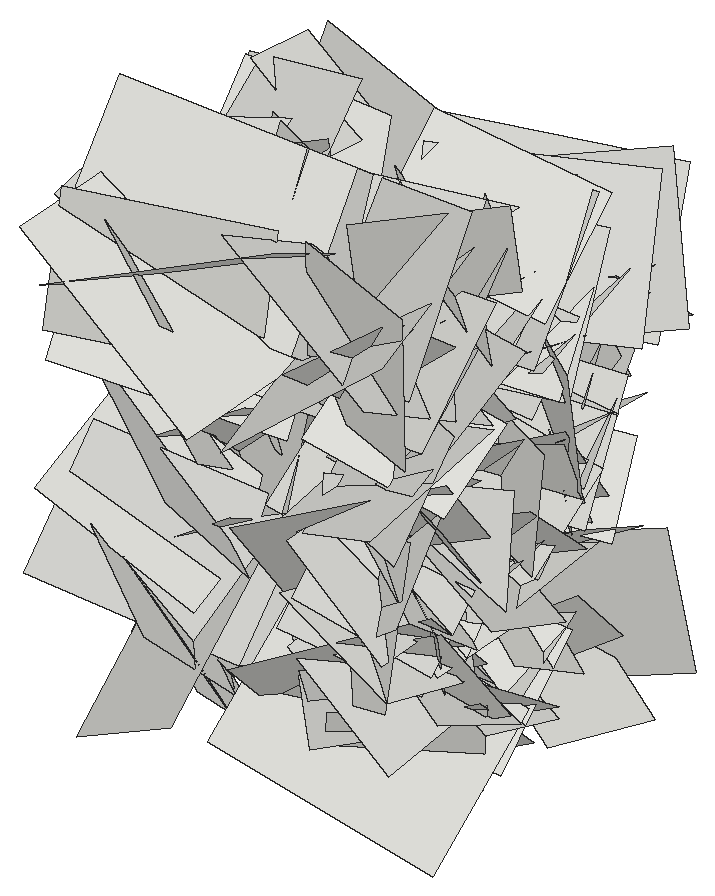
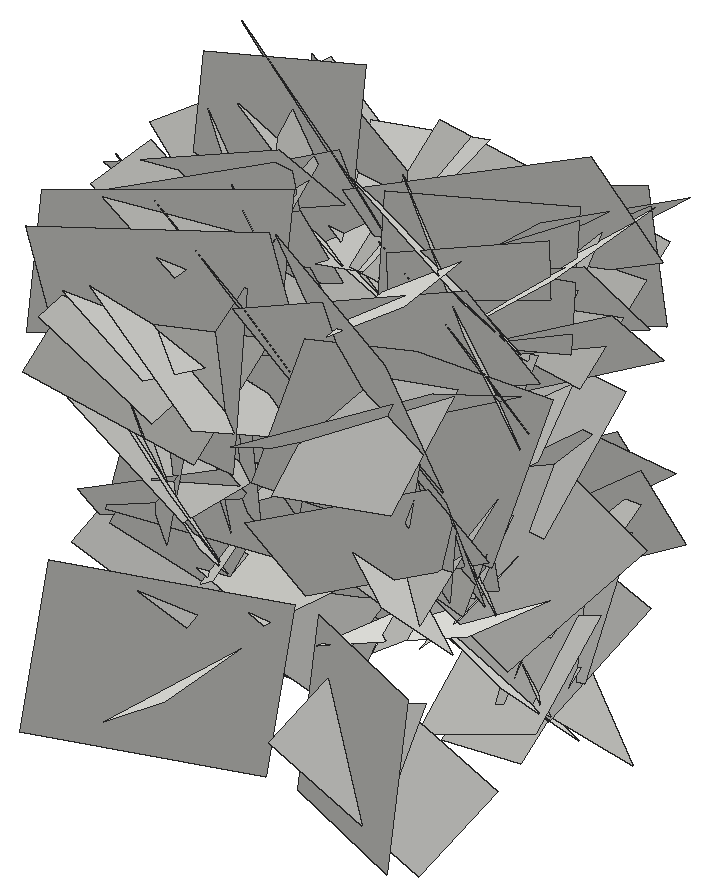
# SketchUp Ruby script. Lengths in inches.
U = 1.inch
M = Sketchup.active_model
def pt(a) = Geom::Point3d.new(a.map { |v| v * U })
def face(e, loops, mat)
  f = e.add_face(loops[0].map { |a| pt(a) })
  loops[1..].each { |l| e.add_face(l.map { |a| pt(a) }).erase! }
  f.material = f.back_material = mat if mat
  f
end
# faces: each face lists its corners as indices into pts; further lists are holes
def faces(e, pts, list, mat = nil) = list.each { |f| face(e, (f[0].is_a?(Array) ? f : [f]).map { |l| l.map { |i| pts[i] } }, mat) }
# xy, xz, yz: faces in a plane at the given z, y or x. An outline is a flat list of corners, or four numbers for a rectangle; further outlines are holes
def ring(l) = l.size == 4 ? [[l[0], l[1]], [l[2], l[1]], [l[2], l[3]], [l[0], l[3]]] : l.each_slice(2).to_a
def flat(e, list, mat, &to3) = list.each { |f| face(e, (f[0].is_a?(Array) ? f : [f]).map { |l| ring(l).map { |u, v| to3.(u, v) } }, mat) }
def xy(e, z, list, mat = nil) = flat(e, list, mat) { |x, y| [x, y, z] }
def xz(e, y, list, mat = nil) = flat(e, list, mat) { |x, z| [x, y, z] }
def yz(e, x, list, mat = nil) = flat(e, list, mat) { |y, z| [x, y, z] }
def lines(e, pts, list) = list.each { |a, b| e.add_line(pt(pts[a]), pt(pts[b])) }
# prism: a flat outline (further loops are holes) pulled along v
def prism(e, loops, v, mat = nil)
  f = face(e, loops, mat); d = Geom::Vector3d.new(v.map { |x| x * U })
  f.pushpull(f.normal.samedirection?(d) ? d.length : -d.length)
end
def box(e, o, s, mat = nil) = prism(e, [[o, [o[0] + s[0], o[1], o[2]], [o[0] + s[0], o[1] + s[1], o[2]], [o[0], o[1] + s[1], o[2]]]], [0, 0, s[2]], mat)
def at(x, y, z, deg = 0) = Geom::Transformation.translation(pt([x, y, z])) * Geom::Transformation.rotation(ORIGIN, Z_AXIS, deg.degrees)
def axes(o, x, y, z) = Geom::Transformation.new([*x, 0, *y, 0, *z, 0, *pt(o).to_a, 1])
def part(name) = M.definitions.add(name)
# library, detail: a bought-in or finely detailed component or shape, given as its bounding box
def library(name, o, s) = part(name).tap { |d| box(d.entities, o, s) }
def detail(e, o, s) = box(e.add_group.entities, o, s)
def put(e, d, t, mat = nil) = e.add_instance(d, t).tap { |i| i.material = mat if mat }
def group(e, t, mat = nil) = e.add_group.tap { |g| g.transformation = t; g.material = mat if mat }.entities
root = M.entities
c1 = part("Component\#6")
p = [[0.01,0,0],[0,3.24,4.54],[4.32,3.24,4.54],[4.33,0,0]]
faces(c1.entities,p,[[0,1,2,3]])
put(root,c1,axes([410.71,158.35,30.49],[-0.08461,0.81055,-0.03501],[-0.12527,-0.04642,-0.80528],[0.85081,0.07377,-0.12204]))
put(root,c1,axes([414.68,161.79,25.53],[-0.01152,-0.82607,0.19056],[-0.15176,0.18963,0.81386],[-0.88572,-0.02175,-0.14193]))
put(root,c1,axes([414.68,162.32,28.44],[-0.12821,-0.42216,-0.69512],[0.01339,-0.70366,0.42514],[-0.86197,0.05186,0.11]))
put(root,c1,axes([400.91,160.22,28.4],[0.15479,0.80897,-0.76348],[-0.02106,-0.76802,-0.81757],[1.17891,-0.11994,0.08565]))
put(root,c1,axes([414.68,160.22,28.4],[-0.15479,0.80897,-0.76348],[0.02106,-0.76802,-0.81757],[-1.17891,-0.11994,0.08565]))
put(root,c1,axes([410.71,158.39,26.84],[-0.02686,0.84806,0.10272],[-0.17857,0.09579,-0.83237],[0.88773,0.04493,-0.16432]))
put(root,c1,axes([400.91,158.99,33.95],[0.09747,0.08794,1.12692],[0.17247,1.11783,-0.1005],[1.18568,-0.16983,-0.07802]))
put(root,c1,axes([414.68,158.99,33.95],[-0.09747,0.08794,1.12692],[-0.17247,1.11783,-0.1005],[-1.18568,-0.16983,-0.07802]))
put(root,c1,axes([404.88,161.42,33.85],[0.12931,-0.58697,0.4315],[0.06321,0.44408,0.58723],[-0.76963,-0.06214,0.12073]))
put(root,c1,axes([410.71,161.42,33.85],[-0.12931,-0.58697,0.4315],[-0.06321,0.44408,0.58723],[0.76963,-0.06214,0.12073]))
put(root,c1,axes([400.91,158.06,26.05],[0.19995,0.52409,1.06255],[0.00833,1.07535,-0.5318],[1.25583,-0.09057,-0.16565]))
put(root,c1,axes([414.68,158.06,26.05],[-0.19995,0.52409,1.06255],[-0.00833,1.07535,-0.5318],[-1.25583,-0.09057,-0.16565]))
put(root,c1,axes([400.91,157.9,37.93],[0.24747,1.3445,0.30187],[-0.11522,0.32319,-1.35538],[1.4561,-0.20293,-0.15855]))
put(root,c1,axes([414.68,157.9,37.93],[-0.24747,1.3445,0.30187],[0.11522,0.32319,-1.35538],[-1.4561,-0.20293,-0.15855]))
put(root,c1,axes([414.68,157.3125,32.29],[0.25179,1.05256,0.51222],[-0.06429,0.53303,-1.06718],[-1.23914,0.18623,0.15945]))
put(root,c1,axes([414.68,158.45,30.92],[0.16236,0.46297,0.88251],[-0.09478,0.89566,-0.45434],[-1.05211,-0.00924,0.17712]))
put(root,c1,axes([400.91,160.96,32.62],[0.12215,0.75895,-0.88724],[0.014,-0.89234,-0.7616],[1.23753,-0.06482,0.09619]))
put(root,c1,axes([414.68,160.96,32.62],[-0.12215,0.75895,-0.88724],[-0.014,-0.89234,-0.7616],[-1.23753,-0.06482,0.09619]))
put(root,c1,axes([400.91,160.7,27.63],[-0.09928,0.64406,-0.88513],[0.13228,-0.87629,-0.65083],[1.15276,0.15602,-0.00154]))
put(root,c1,axes([414.68,160.7,27.63],[0.09928,0.64406,-0.88513],[-0.13228,-0.87629,-0.65083],[-1.15276,0.15602,-0.00154]))
put(root,c1,axes([410.71,160.06,22.6],[-0.02839,-0.24478,0.77995],[-0.15528,0.76918,0.23637],[0.85248,0.13195,0.06903]))
put(root,c1,axes([400.91,164.92,23.28],[0.02573,-1.02703,-0.88101],[-0.12942,-0.87922,1.02158],[1.42847,-0.06116,0.10843]))
put(root,c1,axes([414.68,164.92,23.28],[-0.02573,-1.02703,-0.88101],[0.12942,-0.87922,1.02158],[-1.42847,-0.06116,0.10843]))
put(root,c1,axes([410.71,159.46,22.85],[-0.09982,-0.0635,0.89488],[-0.1784,0.88507,0.04509],[0.93408,0.16225,0.10424]))
put(root,c1,axes([400.91,158.58,28.72],[0.17742,0.80309,0.64454],[-0.10421,0.66248,-0.79991],[1.08655,-0.0676,-0.18196]))
put(root,c1,axes([414.68,158.58,28.72],[-0.17742,0.80309,0.64454],[0.10421,0.66248,-0.79991],[-1.08655,-0.0676,-0.18196]))
put(root,c1,axes([414.68,162.92,24.26],[-0.16568,0.16434,-0.80239],[0.1251,-0.80382,-0.18763],[-0.85913,-0.14874,0.12742]))
put(root,c1,axes([400.91,163.2,33.68],[0.16473,-1.2102,0.57798],[0.2383,0.59712,1.18983],[1.40149,0.04071,-0.27024]))
put(root,c1,axes([414.68,163.2,33.68],[-0.16473,-1.2102,0.57798],[-0.2383,0.59712,1.18983],[-1.40149,0.04071,-0.27024]))
put(root,c1,axes([414.68,163.85,33.45],[0.03445,-0.73428,-0.4148],[-0.17499,-0.41262,0.71747],[-0.87664,0.05351,-0.15952]))
put(root,c1,axes([414.68,162.43,26.35],[-0.02315,-0.70596,0.51236],[0.01203,0.51225,0.70629],[-0.92456,0.02434,-0.00364]))
put(root,c1,axes([414.68,162.61,28.57],[0.04222,-0.49534,0.62953],[-0.20196,0.60636,0.48917],[-0.82474,-0.17384,-0.08755]))
put(root,c1,axes([410.71,162.33,29.83],[-0.22776,0.38392,-0.75072],[0.01782,-0.77261,-0.39993],[0.89361,0.11326,-0.18337]))
put(root,c1,axes([414.68,164.2,31.01],[0.06613,-0.18181,-0.96198],[-0.02897,-0.96387,0.1804],[-1.03734,0.01533,-0.06637]))
put(root,c1,axes([410.71,159.67,28.14],[-0.12868,0.67272,0.52517],[-0.08613,0.51893,-0.68352],[0.90053,0.14576,0.00967]))
put(root,c1,axes([404.88,163.13,28.77],[0.13219,-0.55975,0.33448],[0.05965,0.34851,0.56225],[-0.68862,-0.07726,0.11291]))
put(root,c1,axes([410.71,163.13,28.77],[-0.13219,-0.55975,0.33448],[-0.05965,0.34851,0.56225],[0.68862,-0.07726,0.11291]))
put(root,c1,axes([400.91,159.18,36.25],[0.04304,0.74935,1.15311],[0.14712,1.14549,-0.74928],[1.45028,-0.13844,0.04179]))
put(root,c1,axes([414.68,159.18,36.25],[-0.04304,0.74935,1.15311],[-0.14712,1.14549,-0.74928],[-1.45028,-0.13844,0.04179]))
put(root,c1,axes([410.71,164.96,33.58],[0.03363,-0.67551,-0.53197],[-0.14584,-0.52946,0.66412],[0.89967,-0.06058,0.12754]))
put(root,c1,axes([400.91,159.8,34.2],[-0.03301,0.77795,0.85676],[0.24326,0.8442,-0.75821],[1.20233,-0.14944,0.17692]))
put(root,c1,axes([414.68,159.8,34.2],[0.03301,0.77795,0.85676],[-0.24326,0.8442,-0.75821],[-1.20233,-0.14944,0.17692]))
put(root,c1,axes([414.68,164.8,26.41],[-0.06555,-0.88967,-0.10275],[0.1194,-0.1099,0.88381],[-0.94178,0.04799,0.1192]))
put(root,c1,axes([414.68,163.99,40.83],[-0.08038,0.23372,-0.81219],[0.10222,-0.80774,-0.24144],[-0.89001,-0.11388,0.04562]))
put(root,c1,axes([400.91,162.55,24.47],[0.08094,0.6993,-0.63815],[0.06519,-0.64254,-0.69674],[1.00139,-0.01469,0.09694]))
put(root,c1,axes([414.68,162.55,24.47],[-0.08094,0.6993,-0.63815],[-0.06519,-0.64254,-0.69674],[-1.00139,-0.01469,0.09694]))
put(root,c1,axes([400.91,164.67,22.86],[-0.07455,-1.03669,0.46758],[0.01691,0.46753,1.03897],[1.20537,-0.07068,0.01434]))
put(root,c1,axes([414.68,164.67,22.86],[0.07455,-1.03669,0.46758],[-0.01691,0.46753,1.03897],[-1.20537,-0.07068,0.01434]))
put(root,c1,axes([400.91,159.15,32.85],[-0.28722,0.93511,0.86971],[-0.00467,0.88838,-0.95656],[1.35365,0.20148,0.18123]))
put(root,c1,axes([414.68,159.15,32.85],[0.28722,0.93511,0.86971],[0.00467,0.88838,-0.95656],[-1.35365,0.20148,0.18123]))
put(root,c1,axes([400.91,159.57,38.3125],[-0.19748,1.37219,0.09956],[-0.15298,0.08042,-1.37849],[1.4503,0.19533,-0.13185]))
put(root,c1,axes([414.68,159.57,38.3125],[0.19748,1.37219,0.09956],[0.15298,0.08042,-1.37849],[-1.4503,0.19533,-0.13185]))
put(root,c1,axes([404.88,163.1,21.29],[0.03251,-0.459,0.52355],[0.17075,0.51451,0.44164],[-0.71801,0.10157,0.12873]))
put(root,c1,axes([410.71,163.1,21.29],[-0.03251,-0.459,0.52355],[-0.17075,0.51451,0.44164],[0.71801,0.10157,0.12873]))
put(root,c1,axes([400.91,162.15,25.43],[-0.09766,0.84172,-0.54191],[0.18116,-0.52299,-0.84139],[1.04557,0.16923,0.09516]))
put(root,c1,axes([414.68,162.15,25.43],[0.09766,0.84172,-0.54191],[-0.18116,-0.52299,-0.84139],[-1.04557,0.16923,0.09516]))
put(root,c1,axes([404.88,163.79,31.02],[0.0186,-0.39942,0.51021],[0.04828,0.50989,0.39761],[-0.68514,0.02509,0.04187]))
put(root,c1,axes([410.71,163.79,31.02],[-0.0186,-0.39942,0.51021],[-0.04828,0.50989,0.39761],[0.68514,0.02509,0.04187]))
put(root,c1,axes([400.91,166.67,25.47],[-0.29316,-1.18227,0.54308],[0.10516,0.53443,1.21398],[1.37509,-0.29293,0.02294]))
put(root,c1,axes([414.68,166.67,25.47],[0.29316,-1.18227,0.54308],[-0.10516,0.53443,1.21398],[-1.37509,-0.29293,0.02294]))
put(root,c1,axes([400.91,166.97,25.06],[-0.03339,-0.82276,-0.77538],[0.30966,-0.75526,0.78954],[1.15769,0.17829,-0.23355]))
put(root,c1,axes([414.68,166.97,25.06],[0.03339,-0.82276,-0.77538],[-0.30966,-0.75526,0.78954],[-1.15769,0.17829,-0.23355]))
put(root,c1,axes([400.91,163.625,35.04],[0.27654,-0.44632,0.88094],[-0.09901,0.89592,0.48157],[1.04211,0.20356,-0.18801]))
put(root,c1,axes([414.68,163.625,35.04],[-0.27654,-0.44632,0.88094],[0.09901,0.89592,0.48157],[-1.04211,0.20356,-0.18801]))
put(root,c1,axes([414.68,166.33,22.3],[0.05809,-0.87115,0.26873],[-0.09257,0.26296,0.87026],[-0.96191,-0.07791,-0.06752]))
put(root,c1,axes([400.91,168.45,29.92],[0.2904,-0.81126,-1.09363],[-0.15157,-1.12651,0.79984],[1.4354,0.04517,0.30571]))
put(root,c1,axes([414.68,168.45,29.92],[-0.2904,-0.81126,-1.09363],[0.15157,-1.12651,0.79984],[-1.4354,0.04517,0.30571]))
put(root,c1,axes([404.88,165.16,26.22],[-0.00662,-0.41647,0.48084],[0.04981,0.47925,0.41571],[-0.67246,0.0396,0.02606]))
put(root,c1,axes([410.71,165.16,26.22],[0.00662,-0.41647,0.48084],[-0.04981,0.47925,0.41571],[0.67246,0.0396,0.02606]))
put(root,c1,axes([404.88,165.91,24.52],[-0.03596,-0.58924,0.24858],[0.15481,0.23521,0.57749],[-0.65999,0.08727,0.12191]))
put(root,c1,axes([410.71,165.91,24.52],[0.03596,-0.58924,0.24858],[-0.15481,0.23521,0.57749],[0.65999,0.08727,0.12191]))
put(root,c1,axes([404.88,167.47,38.84],[0.19203,-0.25676,-0.78485],[0.09527,-0.79261,0.28005],[-0.87013,-0.14344,-0.14255]))
put(root,c1,axes([410.71,167.47,38.84],[-0.19203,-0.25676,-0.78485],[-0.09527,-0.79261,0.28005],[0.87013,-0.14344,-0.14255]))
put(root,c1,axes([400.91,168.75,37.98],[-0.06882,-0.53698,-1.12739],[-0.1022,-1.12338,0.54063],[1.31971,-0.115,-0.01692]))
put(root,c1,axes([414.68,168.75,37.98],[0.06882,-0.53698,-1.12739],[0.1022,-1.12338,0.54063],[-1.31971,-0.115,-0.01692]))
put(root,c1,axes([414.68,164.95,29.96],[0.04265,0.57286,-0.52342],[-0.15347,-0.50938,-0.56862],[-0.80809,0.12697,0.08036]))
put(root,c1,axes([414.68,167.29,35.58],[-0.17595,-0.29467,-0.74084],[-0.05215,-0.7515,0.30993],[-0.84352,0.10793,0.13537]))
put(root,c1,axes([410.71,167.69,34.89],[0.01272,-0.59445,-0.3878],[0.01652,-0.38754,0.59453],[0.75216,0.01856,-0.0065]))
put(root,c1,axes([414.68,168.37,37.02],[0.06582,-0.55881,-0.84289],[-0.17414,-0.83883,0.54402],[-1.05774,0.10333,-0.14201]))
put(root,c1,axes([400.91,168.37,37.02],[-0.06582,-0.55881,-0.84289],[0.17414,-0.83883,0.54402],[1.05774,0.10333,-0.14201]))
put(root,c1,axes([400.91,163.85,26.9],[0.03329,1.04875,0.11229],[0.24045,0.10299,-1.02538],[1.09187,-0.05466,0.22238]))
put(root,c1,axes([414.68,163.85,26.9],[-0.03329,1.04875,0.11229],[-0.24045,0.10299,-1.02538],[-1.09187,-0.05466,0.22238]))
put(root,c1,axes([410.71,168.18,25.35],[0.0356,-0.79141,-0.13903],[-0.13499,-0.14264,0.78117],[0.84098,0.01061,0.13127]))
put(root,c1,axes([414.68,164.5,23.79],[-0.04443,0.667,0.37408],[-0.11412,0.36576,-0.66423],[-0.80255,-0.08894,0.07374]))
put(root,c1,axes([400.91,166.55,31.56],[0.0814,0.41102,-0.8284],[0.17089,-0.82447,-0.39413],[0.96524,0.11131,0.13964]))
put(root,c1,axes([414.68,166.55,31.56],[-0.0814,0.41102,-0.8284],[-0.17089,-0.82447,-0.39413],[-0.96524,0.11131,0.13964]))
put(root,c1,axes([400.91,166.62,31.96],[0.21061,0.75098,-0.921],[-0.02022,-0.93165,-0.76377],[1.25951,-0.14053,0.14175]))
put(root,c1,axes([414.68,166.62,31.96],[-0.21061,0.75098,-0.921],[0.02022,-0.93165,-0.76377],[-1.25951,-0.14053,0.14175]))
put(root,c1,axes([414.68,165.04,27.71],[0.04822,0.07219,0.94774],[-0.14201,0.93984,-0.06516],[-0.99746,-0.13032,0.05509]))
put(root,c1,axes([414.68,167.51,23.32],[0.04127,-0.8056,0.43064],[0.05085,0.43224,0.80425],[-0.96695,-0.01165,0.06068]))
put(root,c1,axes([400.91,168.84,39.14],[0.0295,-0.69575,-0.73723],[0.22295,-0.71749,0.68506],[1.05113,0.17171,-0.12461]))
put(root,c1,axes([414.68,168.84,39.14],[-0.0295,-0.69575,-0.73723],[-0.22295,-0.71749,0.68506],[-1.05113,0.17171,-0.12461]))
put(root,c1,axes([410.71,168.23,31.98],[-0.11552,-0.73847,0.10601],[0.00435,0.10653,0.74638],[0.79079,-0.10846,0.01138]))
put(root,c1,axes([404.88,168.24,29.62],[0.00844,-0.1319,-0.59476],[0.00779,-0.59475,0.132],[-0.64572,-0.0089,-0.00618]))
put(root,c1,axes([410.71,168.24,29.62],[-0.00844,-0.1319,-0.59476],[-0.00779,-0.59475,0.132],[0.64572,-0.0089,-0.00618]))
put(root,c1,axes([400.91,169.63,32.59],[0.01533,-0.4611,-1.03377],[0.17767,-1.02158,0.45801],[1.18663,0.15892,-0.05522]))
put(root,c1,axes([414.68,169.63,32.59],[-0.01533,-0.4611,-1.03377],[-0.17767,-1.02158,0.45801],[-1.18663,0.15892,-0.05522]))
put(root,c1,axes([410.71,169.17,27.35],[0.00515,-0.4485,-0.48712],[0.04455,-0.48594,0.44784],[0.70046,0.0342,-0.02491]))
put(root,c1,axes([414.68,171.21,38.93],[0.24063,-0.51313,-1.11059],[0.16085,-1.10901,0.54342],[-1.28679,-0.23458,-0.13976]))
put(root,c1,axes([400.91,169.13,31.47],[0.22896,-0.22184,-0.76377],[0.12794,-0.77313,0.25869],[0.83329,0.17965,0.17014]))
put(root,c1,axes([414.68,169.13,31.47],[-0.22896,-0.22184,-0.76377],[-0.12794,-0.77313,0.25869],[-0.83329,0.17965,0.17014]))
put(root,c1,axes([404.88,168.14,25.37],[0.00005,-0.54267,0.44601],[0.16088,0.43548,0.52984],[-0.72699,0.09633,0.11728]))
put(root,c1,axes([410.71,168.14,25.37],[-0.00005,-0.54267,0.44601],[-0.16088,0.43548,0.52984],[0.72699,0.09633,0.11728]))
put(root,c1,axes([400.91,165.11,34.6875],[0.03998,0.77126,1.05992],[0.2457,1.03973,-0.76482],[1.36759,-0.20934,0.10642]))
put(root,c1,axes([414.68,165.11,34.6875],[-0.03998,0.77126,1.05992],[-0.2457,1.03973,-0.76482],[-1.36759,-0.20934,0.10642]))
put(root,c1,axes([404.88,167.3,30.05],[0.09755,-0.36279,0.79394],[0.2327,0.7823,0.33203],[-0.89554,0.16375,0.17276]))
put(root,c1,axes([410.71,167.3,30.05],[-0.09755,-0.36279,0.79394],[-0.2327,0.7823,0.33203],[0.89554,0.16375,0.17276]))
put(root,c1,axes([400.91,167.41,29.34],[-0.20833,-0.42173,1.22713],[0.0869,1.23461,0.43743],[1.37269,-0.14217,0.15855]))
put(root,c1,axes([414.68,167.41,29.34],[0.20833,-0.42173,1.22713],[-0.0869,1.23461,0.43743],[-1.37269,-0.14217,0.15855]))
put(root,c1,axes([414.68,166.53,31.68],[0.02185,0.89564,-0.0065],[-0.05171,-0.00537,-0.89456],[-0.948,0.02094,0.04865]))
put(root,c1,axes([410.71,169.82,24.93],[0.00586,-0.68753,0.27068],[0.05817,0.27032,0.6855],[0.78107,-0.01497,-0.05308]))
put(root,c1,axes([410.71,169.92,30.86],[0.08798,0.07784,-0.70174],[-0.08853,-0.70052,-0.08758],[0.74315,-0.09267,0.07264]))
put(root,c1,axes([414.68,171.77,39.47],[0.25632,-0.1505,-1.28885],[0.2021,-1.29268,0.18672],[-1.36053,-0.22038,-0.21508]))
put(root,c1,axes([414.68,165.55,34.43],[0.04885,1.13911,0.54464],[-0.08516,0.54654,-1.13629],[-1.33566,0.00681,0.09237]))
put(root,c1,axes([400.91,165.55,34.43],[-0.04885,1.13911,0.54464],[0.08516,0.54654,-1.13629],[1.33566,0.00681,0.09237]))
put(root,c1,axes([404.88,169.1,21.1],[0.05323,-0.42134,0.48328],[0.06346,0.48572,0.41725],[-0.67666,0.01241,0.07715]))
put(root,c1,axes([410.71,169.1,21.1],[-0.05323,-0.42134,0.48328],[-0.06346,0.48572,0.41725],[0.67666,0.01241,0.07715]))
put(root,c1,axes([404.88,170.38,37.22],[0.01844,-0.65259,0.06973],[0.0154,0.07012,0.65262],[-0.69551,-0.01575,0.0163]))
put(root,c1,axes([410.71,170.38,37.22],[-0.01844,-0.65259,0.06973],[-0.0154,0.07012,0.65262],[0.69551,-0.01575,0.0163]))
put(root,c1,axes([404.88,166.74,28.03],[0.20581,0.5378,0.53941],[-0.0447,0.5634,-0.54654],[-0.80617,0.10606,0.16802]))
put(root,c1,axes([410.71,166.74,28.03],[-0.20581,0.5378,0.53941],[0.0447,0.5634,-0.54654],[0.80617,0.10606,0.16802]))
put(root,c1,axes([400.91,170.89,20.28],[0.12274,-1.02279,0.17958],[-0.0333,0.17716,1.02926],[1.10024,0.11946,0.01112]))
put(root,c1,axes([414.68,170.89,20.28],[-0.12274,-1.02279,0.17958],[0.0333,0.17716,1.02926],[-1.10024,0.11946,0.01112]))
put(root,c1,axes([410.71,171.89,34.33],[-0.10287,-0.74562,-0.1631],[0.15609,-0.17961,0.73351],[0.79385,-0.06131,-0.16536]))
put(root,c1,axes([400.91,172.54,38.57],[-0.12011,-0.4932,-1.18141],[0.20578,-1.17893,0.47355],[1.34134,0.1367,-0.17844]))
put(root,c1,axes([414.68,172.54,38.57],[0.12011,-0.4932,-1.18141],[-0.20578,-1.17893,0.47355],[-1.34134,0.1367,-0.17844]))
put(root,c1,axes([400.91,167.53,29.6],[0.04916,0.6172,0.8297],[0.08211,0.82613,-0.61887],[1.09305,-0.08981,0.00917]))
put(root,c1,axes([414.68,167.53,29.6],[-0.04916,0.6172,0.8297],[-0.08211,0.82613,-0.61887],[-1.09305,-0.08981,0.00917]))
put(root,c1,axes([400.91,169.04,36.23],[-0.04162,0.78981,-0.64322],[0.24351,-0.62024,-0.77563],[1.05189,0.17484,0.15411]))
put(root,c1,axes([414.68,169.04,36.23],[0.04162,0.78981,-0.64322],[-0.24351,-0.62024,-0.77563],[-1.05189,0.17484,0.15411]))
put(root,c1,axes([400.91,171.44,26.6],[-0.03428,0.27698,-1.26013],[0.06702,-1.25867,-0.27828],[1.36598,0.0687,-0.01797]))
put(root,c1,axes([414.68,171.44,26.6],[0.03428,0.27698,-1.26013],[-0.06702,-1.25867,-0.27828],[-1.36598,0.0687,-0.01797]))
put(root,c1,axes([410.71,171.91,32.4],[0.07209,-0.36069,-0.54144],[-0.07785,-0.54516,0.35394],[0.6852,-0.024,0.09718]))
put(root,c1,axes([414.68,168.875,35.8],[-0.07444,0.7996,-0.0855],[-0.00091,-0.0859,-0.80263],[-0.85241,-0.06974,0.00832]))
